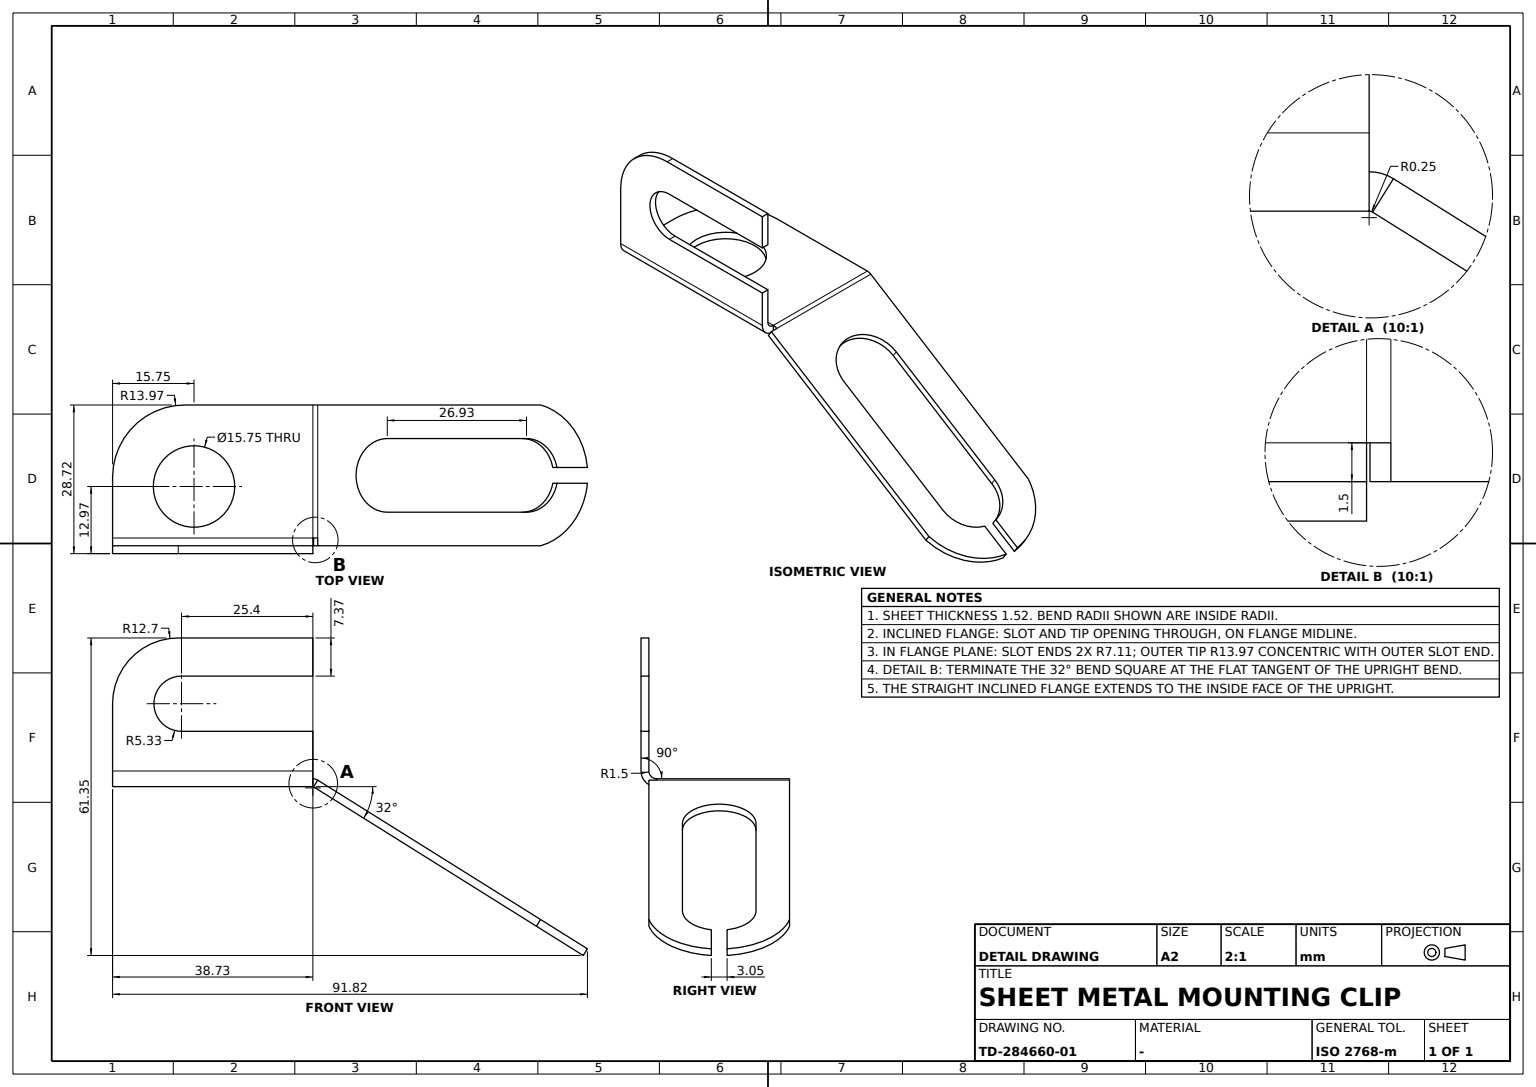
ISO-10303-21;
HEADER;
FILE_DESCRIPTION((''),'2;1');
FILE_NAME('','',(''),(''),'','','');
FILE_SCHEMA(('AUTOMOTIVE_DESIGN'));
ENDSEC;
DATA;
#1=APPLICATION_CONTEXT('');
#2=PRODUCT_CONTEXT('',#1,'mechanical');
#3=PRODUCT('','','',(#2));
#4=PRODUCT_DEFINITION_FORMATION('','',#3);
#5=PRODUCT_DEFINITION_CONTEXT('',#1,'design');
#6=PRODUCT_DEFINITION('','',#4,#5);
#7=PRODUCT_DEFINITION_SHAPE('','',#6);
#8=(LENGTH_UNIT()NAMED_UNIT(*)SI_UNIT(.MILLI.,.METRE.));
#9=(NAMED_UNIT(*)PLANE_ANGLE_UNIT()SI_UNIT($,.RADIAN.));
#10=(NAMED_UNIT(*)SI_UNIT($,.STERADIAN.)SOLID_ANGLE_UNIT());
#11=UNCERTAINTY_MEASURE_WITH_UNIT(LENGTH_MEASURE(0.005),#8,'distance_accuracy_value','');
#12=(GEOMETRIC_REPRESENTATION_CONTEXT(3)GLOBAL_UNCERTAINTY_ASSIGNED_CONTEXT((#11))GLOBAL_UNIT_ASSIGNED_CONTEXT((#8,#9,#10))REPRESENTATION_CONTEXT('',''));
#13=CARTESIAN_POINT('',(72.417726,1.524,-32.856272));
#14=VERTEX_POINT('',#13);
#15=CARTESIAN_POINT('',(63.358061,13.5977,-27.195165));
#16=VERTEX_POINT('',#15);
#17=CARTESIAN_POINT('',(60.641201,0.,-25.497482));
#18=DIRECTION('',(0.529919264,0.,0.848048096));
#19=DIRECTION('',(0.848048096,0.,-0.529919264));
#20=AXIS2_PLACEMENT_3D('',#17,#18,#19);
#21=CIRCLE('',#20,13.97);
#22=EDGE_CURVE('',#14,#16,#21,.T.);
#23=ORIENTED_EDGE('',*,*,#22,.T.);
#24=CARTESIAN_POINT('',(20.26809,13.5977,-0.269563));
#25=VERTEX_POINT('',#24);
#26=CARTESIAN_POINT('',(50.807597,13.5977,-19.352764));
#27=VECTOR('',#19,1000.);
#28=LINE('',#26,#27);
#29=EDGE_CURVE('',#25,#16,#28,.T.);
#30=ORIENTED_EDGE('',*,*,#29,.F.);
#31=CARTESIAN_POINT('',(20.26809,-12.0977,-0.269563));
#32=VERTEX_POINT('',#31);
#33=CARTESIAN_POINT('',(20.26809,0.,-0.269563));
#34=DIRECTION('',(0.,1.,0.));
#35=VECTOR('',#34,1000.);
#36=LINE('',#33,#35);
#37=EDGE_CURVE('',#32,#25,#36,.T.);
#38=ORIENTED_EDGE('',*,*,#37,.F.);
#39=CARTESIAN_POINT('',(20.26809,-13.5977,-0.269563));
#40=VERTEX_POINT('',#39);
#41=DIRECTION('',(0.,-1.,0.));
#42=VECTOR('',#41,1000.);
#43=LINE('',#33,#42);
#44=EDGE_CURVE('',#32,#40,#43,.T.);
#45=ORIENTED_EDGE('',*,*,#44,.T.);
#46=CARTESIAN_POINT('',(63.358061,-13.5977,-27.195165));
#47=VERTEX_POINT('',#46);
#48=CARTESIAN_POINT('',(50.807597,-13.5977,-19.352764));
#49=LINE('',#48,#27);
#50=EDGE_CURVE('',#40,#47,#49,.T.);
#51=ORIENTED_EDGE('',*,*,#50,.T.);
#52=CARTESIAN_POINT('',(72.417726,-1.524,-32.856272));
#53=VERTEX_POINT('',#52);
#54=EDGE_CURVE('',#47,#53,#21,.T.);
#55=ORIENTED_EDGE('',*,*,#54,.T.);
#56=CARTESIAN_POINT('',(66.532418,-1.524,-29.178723));
#57=VERTEX_POINT('',#56);
#58=CARTESIAN_POINT('',(20.207297,-1.524,-0.231575));
#59=DIRECTION('',(-0.848048096,0.,0.529919264));
#60=VECTOR('',#59,1000.);
#61=LINE('',#58,#60);
#62=EDGE_CURVE('',#53,#57,#61,.T.);
#63=ORIENTED_EDGE('',*,*,#62,.T.);
#64=CARTESIAN_POINT('',(60.641201,-7.112,-25.497482));
#65=VERTEX_POINT('',#64);
#66=CIRCLE('',#20,7.112);
#67=EDGE_CURVE('',#65,#57,#66,.T.);
#68=ORIENTED_EDGE('',*,*,#67,.F.);
#69=CARTESIAN_POINT('',(33.715674,-7.112,-8.672545));
#70=VERTEX_POINT('',#69);
#71=CARTESIAN_POINT('',(47.178437,-7.112,-17.085014));
#72=LINE('',#71,#60);
#73=EDGE_CURVE('',#65,#70,#72,.T.);
#74=ORIENTED_EDGE('',*,*,#73,.T.);
#75=CARTESIAN_POINT('',(33.715674,7.112,-8.672545));
#76=VERTEX_POINT('',#75);
#77=CARTESIAN_POINT('',(33.715674,0.,-8.672545));
#78=AXIS2_PLACEMENT_3D('',#77,#18,#19);
#79=CIRCLE('',#78,7.112);
#80=EDGE_CURVE('',#70,#76,#79,.F.);
#81=ORIENTED_EDGE('',*,*,#80,.T.);
#82=CARTESIAN_POINT('',(60.641201,7.112,-25.497482));
#83=VERTEX_POINT('',#82);
#84=CARTESIAN_POINT('',(20.207297,7.112,-0.231575));
#85=LINE('',#84,#60);
#86=EDGE_CURVE('',#83,#76,#85,.T.);
#87=ORIENTED_EDGE('',*,*,#86,.F.);
#88=CARTESIAN_POINT('',(66.532418,1.524,-29.178723));
#89=VERTEX_POINT('',#88);
#90=EDGE_CURVE('',#89,#83,#66,.T.);
#91=ORIENTED_EDGE('',*,*,#90,.F.);
#92=CARTESIAN_POINT('',(20.207297,1.524,-0.231575));
#93=LINE('',#92,#27);
#94=EDGE_CURVE('',#89,#14,#93,.T.);
#95=ORIENTED_EDGE('',*,*,#94,.T.);
#96=EDGE_LOOP('',(#23,#30,#38,#45,#51,#55,#63,#68,#74,#81,#87,#91,#95));
#97=FACE_BOUND('',#96,.T.);
#98=CARTESIAN_POINT('',(20.207297,0.,-0.231575));
#99=AXIS2_PLACEMENT_3D('',#98,#18,#19);
#100=PLANE('',#99);
#101=ADVANCED_FACE('',(#97),#100,.T.);
#102=CARTESIAN_POINT('',(59.833604,-7.112,-26.789907));
#103=VERTEX_POINT('',#102);
#104=VECTOR('',#18,1000.);
#105=LINE('',#64,#104);
#106=EDGE_CURVE('',#65,#103,#105,.F.);
#107=ORIENTED_EDGE('',*,*,#106,.F.);
#108=ORIENTED_EDGE('',*,*,#67,.T.);
#109=CARTESIAN_POINT('',(65.724821,-1.524,-30.471148));
#110=VERTEX_POINT('',#109);
#111=LINE('',#56,#104);
#112=EDGE_CURVE('',#57,#110,#111,.F.);
#113=ORIENTED_EDGE('',*,*,#112,.T.);
#114=CARTESIAN_POINT('',(59.833604,0.,-26.789907));
#115=AXIS2_PLACEMENT_3D('',#114,#18,#19);
#116=CIRCLE('',#115,7.112);
#117=EDGE_CURVE('',#103,#110,#116,.T.);
#118=ORIENTED_EDGE('',*,*,#117,.F.);
#119=EDGE_LOOP('',(#107,#108,#113,#118));
#120=FACE_BOUND('',#119,.T.);
#121=CYLINDRICAL_SURFACE('',#20,7.112);
#122=ADVANCED_FACE('',(#120),#121,.F.);
#123=CARTESIAN_POINT('',(62.550464,-13.5977,-28.48759));
#124=VERTEX_POINT('',#123);
#125=LINE('',#46,#104);
#126=EDGE_CURVE('',#47,#124,#125,.F.);
#127=ORIENTED_EDGE('',*,*,#126,.T.);
#128=CARTESIAN_POINT('',(71.610129,-1.524,-34.148697));
#129=VERTEX_POINT('',#128);
#130=CIRCLE('',#115,13.97);
#131=EDGE_CURVE('',#124,#129,#130,.T.);
#132=ORIENTED_EDGE('',*,*,#131,.T.);
#133=LINE('',#52,#104);
#134=EDGE_CURVE('',#53,#129,#133,.F.);
#135=ORIENTED_EDGE('',*,*,#134,.F.);
#136=ORIENTED_EDGE('',*,*,#54,.F.);
#137=EDGE_LOOP('',(#127,#132,#135,#136));
#138=FACE_BOUND('',#137,.T.);
#139=CYLINDRICAL_SURFACE('',#20,13.97);
#140=ADVANCED_FACE('',(#138),#139,.T.);
#141=CARTESIAN_POINT('',(-19.3997,-0.3723,0.));
#142=VERTEX_POINT('',#141);
#143=CARTESIAN_POINT('',(-5.4297,13.5977,0.));
#144=VERTEX_POINT('',#143);
#145=CARTESIAN_POINT('',(-5.4297,-0.3723,0.));
#146=DIRECTION('',(0.,0.,-1.));
#147=DIRECTION('',(-1.,0.,0.));
#148=AXIS2_PLACEMENT_3D('',#145,#146,#147);
#149=CIRCLE('',#148,13.97);
#150=EDGE_CURVE('',#142,#144,#149,.T.);
#151=ORIENTED_EDGE('',*,*,#150,.F.);
#152=CARTESIAN_POINT('',(-19.3997,-12.0977,0.));
#153=VERTEX_POINT('',#152);
#154=CARTESIAN_POINT('',(-19.3997,0.,0.));
#155=LINE('',#154,#35);
#156=EDGE_CURVE('',#153,#142,#155,.T.);
#157=ORIENTED_EDGE('',*,*,#156,.F.);
#158=CARTESIAN_POINT('',(19.328014,-12.0977,0.));
#159=VERTEX_POINT('',#158);
#160=CARTESIAN_POINT('',(-0.035843,-12.0977,0.));
#161=DIRECTION('',(1.,0.,0.));
#162=VECTOR('',#161,1000.);
#163=LINE('',#160,#162);
#164=EDGE_CURVE('',#153,#159,#163,.T.);
#165=ORIENTED_EDGE('',*,*,#164,.T.);
#166=CARTESIAN_POINT('',(19.328014,13.5977,0.));
#167=VERTEX_POINT('',#166);
#168=CARTESIAN_POINT('',(19.328014,0.,0.));
#169=LINE('',#168,#35);
#170=EDGE_CURVE('',#159,#167,#169,.T.);
#171=ORIENTED_EDGE('',*,*,#170,.T.);
#172=CARTESIAN_POINT('',(0.,13.5977,0.));
#173=LINE('',#172,#162);
#174=EDGE_CURVE('',#144,#167,#173,.T.);
#175=ORIENTED_EDGE('',*,*,#174,.F.);
#176=EDGE_LOOP('',(#151,#157,#165,#171,#175));
#177=FACE_BOUND('',#176,.T.);
#178=CARTESIAN_POINT('',(-11.5257,-2.1503,0.));
#179=VERTEX_POINT('',#178);
#180=CARTESIAN_POINT('',(-3.6517,-2.1503,0.));
#181=AXIS2_PLACEMENT_3D('',#180,#146,#147);
#182=CIRCLE('',#181,7.874);
#183=EDGE_CURVE('',#179,#179,#182,.T.);
#184=ORIENTED_EDGE('',*,*,#183,.T.);
#185=EDGE_LOOP('',(#184));
#186=FACE_BOUND('',#185,.T.);
#187=CARTESIAN_POINT('',(0.,0.,0.));
#188=AXIS2_PLACEMENT_3D('',#187,#146,#41);
#189=PLANE('',#188);
#190=ADVANCED_FACE('',(#177,#186),#189,.F.);
#191=CARTESIAN_POINT('',(-19.3997,-0.3723,-1.524));
#192=VERTEX_POINT('',#191);
#193=CARTESIAN_POINT('',(-5.4297,13.5977,-1.524));
#194=VERTEX_POINT('',#193);
#195=CARTESIAN_POINT('',(-5.4297,-0.3723,-1.524));
#196=AXIS2_PLACEMENT_3D('',#195,#146,#147);
#197=CIRCLE('',#196,13.97);
#198=EDGE_CURVE('',#192,#194,#197,.T.);
#199=ORIENTED_EDGE('',*,*,#198,.F.);
#200=VECTOR('',#146,1000.);
#201=LINE('',#141,#200);
#202=EDGE_CURVE('',#142,#192,#201,.T.);
#203=ORIENTED_EDGE('',*,*,#202,.F.);
#204=ORIENTED_EDGE('',*,*,#150,.T.);
#205=LINE('',#143,#200);
#206=EDGE_CURVE('',#144,#194,#205,.T.);
#207=ORIENTED_EDGE('',*,*,#206,.T.);
#208=EDGE_LOOP('',(#199,#203,#204,#207));
#209=FACE_BOUND('',#208,.T.);
#210=AXIS2_PLACEMENT_3D('',#145,#146,#41);
#211=CYLINDRICAL_SURFACE('',#210,13.97);
#212=ADVANCED_FACE('',(#209),#211,.T.);
#213=ORIENTED_EDGE('',*,*,#198,.T.);
#214=CARTESIAN_POINT('',(19.328014,13.5977,-1.524));
#215=VERTEX_POINT('',#214);
#216=CARTESIAN_POINT('',(0.,13.5977,-1.524));
#217=LINE('',#216,#162);
#218=EDGE_CURVE('',#194,#215,#217,.T.);
#219=ORIENTED_EDGE('',*,*,#218,.T.);
#220=CARTESIAN_POINT('',(19.328014,-12.0977,-1.524));
#221=VERTEX_POINT('',#220);
#222=CARTESIAN_POINT('',(19.328014,0.,-1.524));
#223=LINE('',#222,#35);
#224=EDGE_CURVE('',#221,#215,#223,.T.);
#225=ORIENTED_EDGE('',*,*,#224,.F.);
#226=CARTESIAN_POINT('',(-19.3997,-12.0977,-1.524));
#227=VERTEX_POINT('',#226);
#228=CARTESIAN_POINT('',(-0.035843,-12.0977,-1.524));
#229=LINE('',#228,#162);
#230=EDGE_CURVE('',#227,#221,#229,.T.);
#231=ORIENTED_EDGE('',*,*,#230,.F.);
#232=CARTESIAN_POINT('',(-19.3997,0.,-1.524));
#233=LINE('',#232,#35);
#234=EDGE_CURVE('',#227,#192,#233,.T.);
#235=ORIENTED_EDGE('',*,*,#234,.T.);
#236=EDGE_LOOP('',(#213,#219,#225,#231,#235));
#237=FACE_BOUND('',#236,.T.);
#238=CARTESIAN_POINT('',(-11.5257,-2.1503,-1.524));
#239=VERTEX_POINT('',#238);
#240=CARTESIAN_POINT('',(-3.6517,-2.1503,-1.524));
#241=AXIS2_PLACEMENT_3D('',#240,#146,#147);
#242=CIRCLE('',#241,7.874);
#243=EDGE_CURVE('',#239,#239,#242,.T.);
#244=ORIENTED_EDGE('',*,*,#243,.F.);
#245=EDGE_LOOP('',(#244));
#246=FACE_BOUND('',#245,.T.);
#247=CARTESIAN_POINT('',(0.,0.,-1.524));
#248=AXIS2_PLACEMENT_3D('',#247,#146,#41);
#249=PLANE('',#248);
#250=ADVANCED_FACE('',(#237,#246),#249,.T.);
#251=ORIENTED_EDGE('',*,*,#206,.F.);
#252=ORIENTED_EDGE('',*,*,#174,.T.);
#253=CARTESIAN_POINT('',(19.328014,13.5977,-1.774));
#254=DIRECTION('',(0.,0.,1.));
#255=AXIS2_PLACEMENT_3D('',#253,#34,#254);
#256=CIRCLE('',#255,1.774);
#257=EDGE_CURVE('',#25,#167,#256,.F.);
#258=ORIENTED_EDGE('',*,*,#257,.F.);
#259=ORIENTED_EDGE('',*,*,#29,.T.);
#260=CARTESIAN_POINT('',(62.550464,13.5977,-28.48759));
#261=VERTEX_POINT('',#260);
#262=LINE('',#15,#104);
#263=EDGE_CURVE('',#16,#261,#262,.F.);
#264=ORIENTED_EDGE('',*,*,#263,.T.);
#265=CARTESIAN_POINT('',(19.460493,13.5977,-1.561988));
#266=VERTEX_POINT('',#265);
#267=CARTESIAN_POINT('',(50.,13.5977,-20.64519));
#268=LINE('',#267,#27);
#269=EDGE_CURVE('',#266,#261,#268,.T.);
#270=ORIENTED_EDGE('',*,*,#269,.F.);
#271=CIRCLE('',#255,0.25);
#272=EDGE_CURVE('',#266,#215,#271,.F.);
#273=ORIENTED_EDGE('',*,*,#272,.T.);
#274=ORIENTED_EDGE('',*,*,#218,.F.);
#275=EDGE_LOOP('',(#251,#252,#258,#259,#264,#270,#273,#274));
#276=FACE_BOUND('',#275,.T.);
#277=CARTESIAN_POINT('',(50.403798,13.5977,-19.998977));
#278=AXIS2_PLACEMENT_3D('',#277,#34,#161);
#279=PLANE('',#278);
#280=ADVANCED_FACE('',(#276),#279,.T.);
#281=CARTESIAN_POINT('',(19.328014,-13.5977,27.1984));
#282=VERTEX_POINT('',#281);
#283=CARTESIAN_POINT('',(-6.6997,-13.5977,27.1984));
#284=VERTEX_POINT('',#283);
#285=CARTESIAN_POINT('',(50.403798,-13.5977,27.1984));
#286=VECTOR('',#147,1000.);
#287=LINE('',#285,#286);
#288=EDGE_CURVE('',#282,#284,#287,.T.);
#289=ORIENTED_EDGE('',*,*,#288,.F.);
#290=CARTESIAN_POINT('',(19.328014,-13.5977,19.8324));
#291=VERTEX_POINT('',#290);
#292=LINE('',#281,#200);
#293=EDGE_CURVE('',#282,#291,#292,.T.);
#294=ORIENTED_EDGE('',*,*,#293,.T.);
#295=CARTESIAN_POINT('',(-6.071986,-13.5977,19.8324));
#296=VERTEX_POINT('',#295);
#297=LINE('',#290,#286);
#298=EDGE_CURVE('',#291,#296,#297,.T.);
#299=ORIENTED_EDGE('',*,*,#298,.T.);
#300=CARTESIAN_POINT('',(-6.071986,-13.5977,9.1644));
#301=VERTEX_POINT('',#300);
#302=CARTESIAN_POINT('',(-6.071986,-13.5977,14.4984));
#303=AXIS2_PLACEMENT_3D('',#302,#34,#254);
#304=CIRCLE('',#303,5.334);
#305=EDGE_CURVE('',#301,#296,#304,.T.);
#306=ORIENTED_EDGE('',*,*,#305,.F.);
#307=CARTESIAN_POINT('',(19.328014,-13.5977,9.1644));
#308=VERTEX_POINT('',#307);
#309=CARTESIAN_POINT('',(50.403798,-13.5977,9.1644));
#310=LINE('',#309,#286);
#311=EDGE_CURVE('',#308,#301,#310,.T.);
#312=ORIENTED_EDGE('',*,*,#311,.F.);
#313=CARTESIAN_POINT('',(19.328014,-13.5977,1.5));
#314=VERTEX_POINT('',#313);
#315=CARTESIAN_POINT('',(19.328014,-13.5977,-19.998977));
#316=VECTOR('',#254,1000.);
#317=LINE('',#315,#316);
#318=EDGE_CURVE('',#314,#308,#317,.T.);
#319=ORIENTED_EDGE('',*,*,#318,.F.);
#320=CARTESIAN_POINT('',(-19.3997,-13.5977,1.5));
#321=VERTEX_POINT('',#320);
#322=CARTESIAN_POINT('',(-0.035843,-13.5977,1.5));
#323=LINE('',#322,#162);
#324=EDGE_CURVE('',#321,#314,#323,.T.);
#325=ORIENTED_EDGE('',*,*,#324,.F.);
#326=CARTESIAN_POINT('',(-19.3997,-13.5977,14.4984));
#327=VERTEX_POINT('',#326);
#328=CARTESIAN_POINT('',(-19.3997,-13.5977,-19.998977));
#329=LINE('',#328,#316);
#330=EDGE_CURVE('',#327,#321,#329,.F.);
#331=ORIENTED_EDGE('',*,*,#330,.F.);
#332=CARTESIAN_POINT('',(-6.6997,-13.5977,14.4984));
#333=AXIS2_PLACEMENT_3D('',#332,#34,#254);
#334=CIRCLE('',#333,12.7);
#335=EDGE_CURVE('',#284,#327,#334,.F.);
#336=ORIENTED_EDGE('',*,*,#335,.F.);
#337=EDGE_LOOP('',(#289,#294,#299,#306,#312,#319,#325,#331,#336));
#338=FACE_BOUND('',#337,.T.);
#339=CARTESIAN_POINT('',(50.403798,-13.5977,-19.998977));
#340=AXIS2_PLACEMENT_3D('',#339,#34,#161);
#341=PLANE('',#340);
#342=ADVANCED_FACE('',(#338),#341,.T.);
#343=CARTESIAN_POINT('',(19.460493,-12.0977,-1.561988));
#344=VERTEX_POINT('',#343);
#345=CARTESIAN_POINT('',(19.328014,-12.0977,-1.774));
#346=AXIS2_PLACEMENT_3D('',#345,#41,#146);
#347=CIRCLE('',#346,0.25);
#348=EDGE_CURVE('',#344,#221,#347,.T.);
#349=ORIENTED_EDGE('',*,*,#348,.T.);
#350=ORIENTED_EDGE('',*,*,#224,.T.);
#351=ORIENTED_EDGE('',*,*,#272,.F.);
#352=CARTESIAN_POINT('',(19.460493,0.,-1.561988));
#353=LINE('',#352,#35);
#354=EDGE_CURVE('',#344,#266,#353,.T.);
#355=ORIENTED_EDGE('',*,*,#354,.F.);
#356=EDGE_LOOP('',(#349,#350,#351,#355));
#357=FACE_BOUND('',#356,.T.);
#358=CARTESIAN_POINT('',(19.328014,0.,-1.774));
#359=AXIS2_PLACEMENT_3D('',#358,#34,#254);
#360=CYLINDRICAL_SURFACE('',#359,0.25);
#361=ADVANCED_FACE('',(#357),#360,.F.);
#362=LINE('',#158,#200);
#363=EDGE_CURVE('',#159,#221,#362,.T.);
#364=ORIENTED_EDGE('',*,*,#363,.T.);
#365=ORIENTED_EDGE('',*,*,#348,.F.);
#366=DIRECTION('',(-0.529919264,0.,-0.848048096));
#367=VECTOR('',#366,1000.);
#368=LINE('',#343,#367);
#369=EDGE_CURVE('',#32,#344,#368,.T.);
#370=ORIENTED_EDGE('',*,*,#369,.F.);
#371=CIRCLE('',#346,1.774);
#372=EDGE_CURVE('',#32,#159,#371,.T.);
#373=ORIENTED_EDGE('',*,*,#372,.T.);
#374=EDGE_LOOP('',(#364,#365,#370,#373));
#375=FACE_BOUND('',#374,.T.);
#376=DIRECTION('',(-0.913545458,0.,0.406736643));
#377=AXIS2_PLACEMENT_3D('',#343,#41,#376);
#378=PLANE('',#377);
#379=ADVANCED_FACE('',(#375),#378,.T.);
#380=CARTESIAN_POINT('',(19.460493,-13.5977,-1.561988));
#381=VERTEX_POINT('',#380);
#382=CARTESIAN_POINT('',(50.,-13.5977,-20.64519));
#383=LINE('',#382,#27);
#384=EDGE_CURVE('',#381,#124,#383,.T.);
#385=ORIENTED_EDGE('',*,*,#384,.T.);
#386=ORIENTED_EDGE('',*,*,#126,.F.);
#387=ORIENTED_EDGE('',*,*,#50,.F.);
#388=LINE('',#380,#367);
#389=EDGE_CURVE('',#40,#381,#388,.T.);
#390=ORIENTED_EDGE('',*,*,#389,.T.);
#391=EDGE_LOOP('',(#385,#386,#387,#390));
#392=FACE_BOUND('',#391,.T.);
#393=ADVANCED_FACE('',(#392),#341,.F.);
#394=CARTESIAN_POINT('',(19.328014,-15.1217,1.5));
#395=VERTEX_POINT('',#394);
#396=LINE('',#313,#42);
#397=EDGE_CURVE('',#314,#395,#396,.T.);
#398=ORIENTED_EDGE('',*,*,#397,.F.);
#399=ORIENTED_EDGE('',*,*,#318,.T.);
#400=CARTESIAN_POINT('',(19.328014,-15.1217,9.1644));
#401=VERTEX_POINT('',#400);
#402=LINE('',#307,#35);
#403=EDGE_CURVE('',#401,#308,#402,.T.);
#404=ORIENTED_EDGE('',*,*,#403,.F.);
#405=CARTESIAN_POINT('',(19.328014,-15.1217,0.));
#406=LINE('',#405,#316);
#407=EDGE_CURVE('',#395,#401,#406,.T.);
#408=ORIENTED_EDGE('',*,*,#407,.F.);
#409=EDGE_LOOP('',(#398,#399,#404,#408));
#410=FACE_BOUND('',#409,.T.);
#411=AXIS2_PLACEMENT_3D('',#281,#147,#146);
#412=PLANE('',#411);
#413=ADVANCED_FACE('',(#410),#412,.F.);
#414=ORIENTED_EDGE('',*,*,#243,.T.);
#415=EDGE_LOOP('',(#414));
#416=FACE_BOUND('',#415,.T.);
#417=ORIENTED_EDGE('',*,*,#183,.F.);
#418=EDGE_LOOP('',(#417));
#419=FACE_BOUND('',#418,.T.);
#420=CARTESIAN_POINT('',(-3.6517,-2.1503,-0.762));
#421=AXIS2_PLACEMENT_3D('',#420,#146,#161);
#422=CYLINDRICAL_SURFACE('',#421,7.874);
#423=ADVANCED_FACE('',(#416,#419),#422,.F.);
#424=CARTESIAN_POINT('',(65.724821,1.524,-30.471148));
#425=VERTEX_POINT('',#424);
#426=CARTESIAN_POINT('',(71.610129,1.524,-34.148697));
#427=VERTEX_POINT('',#426);
#428=CARTESIAN_POINT('',(19.3997,1.524,-1.524));
#429=LINE('',#428,#27);
#430=EDGE_CURVE('',#425,#427,#429,.T.);
#431=ORIENTED_EDGE('',*,*,#430,.T.);
#432=LINE('',#13,#104);
#433=EDGE_CURVE('',#14,#427,#432,.F.);
#434=ORIENTED_EDGE('',*,*,#433,.F.);
#435=ORIENTED_EDGE('',*,*,#94,.F.);
#436=LINE('',#88,#104);
#437=EDGE_CURVE('',#89,#425,#436,.F.);
#438=ORIENTED_EDGE('',*,*,#437,.T.);
#439=EDGE_LOOP('',(#431,#434,#435,#438));
#440=FACE_BOUND('',#439,.T.);
#441=CARTESIAN_POINT('',(69.475072,1.524,-31.017497));
#442=AXIS2_PLACEMENT_3D('',#441,#41,#161);
#443=PLANE('',#442);
#444=ADVANCED_FACE('',(#440),#443,.T.);
#445=CARTESIAN_POINT('',(-19.3997,-15.1217,1.5));
#446=VERTEX_POINT('',#445);
#447=LINE('',#320,#35);
#448=EDGE_CURVE('',#321,#446,#447,.F.);
#449=ORIENTED_EDGE('',*,*,#448,.T.);
#450=CARTESIAN_POINT('',(-19.3997,-15.1217,14.4984));
#451=VERTEX_POINT('',#450);
#452=CARTESIAN_POINT('',(-19.3997,-15.1217,0.));
#453=LINE('',#452,#316);
#454=EDGE_CURVE('',#451,#446,#453,.F.);
#455=ORIENTED_EDGE('',*,*,#454,.F.);
#456=LINE('',#326,#35);
#457=EDGE_CURVE('',#327,#451,#456,.F.);
#458=ORIENTED_EDGE('',*,*,#457,.F.);
#459=ORIENTED_EDGE('',*,*,#330,.T.);
#460=EDGE_LOOP('',(#449,#455,#458,#459));
#461=FACE_BOUND('',#460,.T.);
#462=CARTESIAN_POINT('',(-19.3997,-13.5977,0.));
#463=AXIS2_PLACEMENT_3D('',#462,#147,#34);
#464=PLANE('',#463);
#465=ADVANCED_FACE('',(#461),#464,.T.);
#466=CARTESIAN_POINT('',(-0.035843,-15.1217,1.5));
#467=LINE('',#466,#162);
#468=EDGE_CURVE('',#446,#395,#467,.T.);
#469=ORIENTED_EDGE('',*,*,#468,.T.);
#470=ORIENTED_EDGE('',*,*,#407,.T.);
#471=CARTESIAN_POINT('',(-6.071986,-15.1217,9.1644));
#472=VERTEX_POINT('',#471);
#473=CARTESIAN_POINT('',(0.,-15.1217,9.1644));
#474=LINE('',#473,#286);
#475=EDGE_CURVE('',#401,#472,#474,.T.);
#476=ORIENTED_EDGE('',*,*,#475,.T.);
#477=CARTESIAN_POINT('',(-6.071986,-15.1217,19.8324));
#478=VERTEX_POINT('',#477);
#479=CARTESIAN_POINT('',(-6.071986,-15.1217,14.4984));
#480=AXIS2_PLACEMENT_3D('',#479,#34,#254);
#481=CIRCLE('',#480,5.334);
#482=EDGE_CURVE('',#472,#478,#481,.T.);
#483=ORIENTED_EDGE('',*,*,#482,.T.);
#484=CARTESIAN_POINT('',(19.328014,-15.1217,19.8324));
#485=VERTEX_POINT('',#484);
#486=LINE('',#484,#286);
#487=EDGE_CURVE('',#485,#478,#486,.T.);
#488=ORIENTED_EDGE('',*,*,#487,.F.);
#489=CARTESIAN_POINT('',(19.328014,-15.1217,27.1984));
#490=VERTEX_POINT('',#489);
#491=LINE('',#489,#200);
#492=EDGE_CURVE('',#490,#485,#491,.T.);
#493=ORIENTED_EDGE('',*,*,#492,.F.);
#494=CARTESIAN_POINT('',(-6.6997,-15.1217,27.1984));
#495=VERTEX_POINT('',#494);
#496=CARTESIAN_POINT('',(0.,-15.1217,27.1984));
#497=LINE('',#496,#286);
#498=EDGE_CURVE('',#490,#495,#497,.T.);
#499=ORIENTED_EDGE('',*,*,#498,.T.);
#500=CARTESIAN_POINT('',(-6.6997,-15.1217,14.4984));
#501=AXIS2_PLACEMENT_3D('',#500,#34,#254);
#502=CIRCLE('',#501,12.7);
#503=EDGE_CURVE('',#495,#451,#502,.F.);
#504=ORIENTED_EDGE('',*,*,#503,.T.);
#505=ORIENTED_EDGE('',*,*,#454,.T.);
#506=EDGE_LOOP('',(#469,#470,#476,#483,#488,#493,#499,#504,#505));
#507=FACE_BOUND('',#506,.T.);
#508=CARTESIAN_POINT('',(0.,-15.1217,0.));
#509=AXIS2_PLACEMENT_3D('',#508,#34,#147);
#510=PLANE('',#509);
#511=ADVANCED_FACE('',(#507),#510,.F.);
#512=LINE('',#152,#200);
#513=EDGE_CURVE('',#153,#227,#512,.T.);
#514=ORIENTED_EDGE('',*,*,#513,.T.);
#515=CARTESIAN_POINT('',(-19.3997,-12.0977,1.5));
#516=AXIS2_PLACEMENT_3D('',#515,#161,#146);
#517=CIRCLE('',#516,3.024);
#518=EDGE_CURVE('',#446,#227,#517,.T.);
#519=ORIENTED_EDGE('',*,*,#518,.F.);
#520=ORIENTED_EDGE('',*,*,#448,.F.);
#521=CIRCLE('',#516,1.5);
#522=EDGE_CURVE('',#321,#153,#521,.T.);
#523=ORIENTED_EDGE('',*,*,#522,.T.);
#524=EDGE_LOOP('',(#514,#519,#520,#523));
#525=FACE_BOUND('',#524,.T.);
#526=CARTESIAN_POINT('',(-19.3997,-12.239072,0.));
#527=CARTESIAN_POINT('',(-19.3997,-12.382705,-1.524));
#528=CARTESIAN_POINT('',(-19.3997,-12.380443,0.016655));
#529=CARTESIAN_POINT('',(-19.3997,-12.667711,-1.490424));
#530=CARTESIAN_POINT('',(-19.3997,-12.519198,0.049967));
#531=CARTESIAN_POINT('',(-19.3997,-12.947441,-1.423266));
#532=CARTESIAN_POINT('',(-19.3997,-12.786247,0.148651));
#533=CARTESIAN_POINT('',(-19.3997,-13.485811,-1.224321));
#534=CARTESIAN_POINT('',(-19.3997,-13.023051,0.306693));
#535=CARTESIAN_POINT('',(-19.3997,-13.963207,-0.905708));
#536=CARTESIAN_POINT('',(-19.3997,-13.131559,0.399367));
#537=CARTESIAN_POINT('',(-19.3997,-14.18196,-0.718875));
#538=CARTESIAN_POINT('',(-19.3997,-13.3247,0.608533));
#539=CARTESIAN_POINT('',(-19.3997,-14.571331,-0.297198));
#540=CARTESIAN_POINT('',(-19.3997,-13.463944,0.856856));
#541=CARTESIAN_POINT('',(-19.3997,-14.852047,0.203421));
#542=CARTESIAN_POINT('',(-19.3997,-13.518552,0.988691));
#543=CARTESIAN_POINT('',(-19.3997,-14.962137,0.469202));
#544=CARTESIAN_POINT('',(-19.3997,-13.569972,1.171392));
#545=CARTESIAN_POINT('',(-19.3997,-15.065801,0.837527));
#546=CARTESIAN_POINT('',(-19.3997,-13.592148,1.358725));
#547=CARTESIAN_POINT('',(-19.3997,-15.110508,1.21519));
#548=CARTESIAN_POINT('',(-19.3997,-13.595849,1.405752));
#549=CARTESIAN_POINT('',(-19.3997,-15.117969,1.309996));
#550=CARTESIAN_POINT('',(-19.3997,-13.5977,1.452876));
#551=CARTESIAN_POINT('',(-19.3997,-15.1217,1.404998));
#552=B_SPLINE_SURFACE_WITH_KNOTS('',5,1,((#152,#226),(#526,#527),(#528,#529),(#530,#531),(#532,#533),(#534,#535),(#536,#537),(#538,#539),(#540,#541),(#542,#543),(#544,#545),(#546,#547),(#548,#549),(#550,#551),(#320,#445)),.RULED_SURF.,.F.,.F.,.F.,(6,3,3,3,6),(2,2),(0.,0.0045,0.009,0.0135,0.015),(0.,0.0015),.UNSPECIFIED.);
#553=ADVANCED_FACE('',(#525),#552,.F.);
#554=ORIENTED_EDGE('',*,*,#44,.F.);
#555=ORIENTED_EDGE('',*,*,#369,.T.);
#556=LINE('',#352,#42);
#557=EDGE_CURVE('',#344,#381,#556,.T.);
#558=ORIENTED_EDGE('',*,*,#557,.T.);
#559=ORIENTED_EDGE('',*,*,#389,.F.);
#560=EDGE_LOOP('',(#554,#555,#558,#559));
#561=FACE_BOUND('',#560,.T.);
#562=CARTESIAN_POINT('',(19.460493,-12.8477,-1.561988));
#563=AXIS2_PLACEMENT_3D('',#562,#59,#18);
#564=PLANE('',#563);
#565=ADVANCED_FACE('',(#561),#564,.T.);
#566=ORIENTED_EDGE('',*,*,#503,.F.);
#567=LINE('',#283,#35);
#568=EDGE_CURVE('',#284,#495,#567,.F.);
#569=ORIENTED_EDGE('',*,*,#568,.F.);
#570=ORIENTED_EDGE('',*,*,#335,.T.);
#571=ORIENTED_EDGE('',*,*,#457,.T.);
#572=EDGE_LOOP('',(#566,#569,#570,#571));
#573=FACE_BOUND('',#572,.T.);
#574=AXIS2_PLACEMENT_3D('',#332,#34,#147);
#575=CYLINDRICAL_SURFACE('',#574,12.7);
#576=ADVANCED_FACE('',(#573),#575,.T.);
#577=LINE('',#281,#35);
#578=EDGE_CURVE('',#490,#282,#577,.T.);
#579=ORIENTED_EDGE('',*,*,#578,.T.);
#580=ORIENTED_EDGE('',*,*,#288,.T.);
#581=ORIENTED_EDGE('',*,*,#568,.T.);
#582=ORIENTED_EDGE('',*,*,#498,.F.);
#583=EDGE_LOOP('',(#579,#580,#581,#582));
#584=FACE_BOUND('',#583,.T.);
#585=CARTESIAN_POINT('',(-19.3997,-13.5977,27.1984));
#586=AXIS2_PLACEMENT_3D('',#585,#146,#161);
#587=PLANE('',#586);
#588=ADVANCED_FACE('',(#584),#587,.F.);
#589=ORIENTED_EDGE('',*,*,#90,.T.);
#590=CARTESIAN_POINT('',(59.833604,7.112,-26.789907));
#591=VERTEX_POINT('',#590);
#592=LINE('',#82,#104);
#593=EDGE_CURVE('',#83,#591,#592,.F.);
#594=ORIENTED_EDGE('',*,*,#593,.T.);
#595=EDGE_CURVE('',#425,#591,#116,.T.);
#596=ORIENTED_EDGE('',*,*,#595,.F.);
#597=ORIENTED_EDGE('',*,*,#437,.F.);
#598=EDGE_LOOP('',(#589,#594,#596,#597));
#599=FACE_BOUND('',#598,.T.);
#600=ADVANCED_FACE('',(#599),#121,.F.);
#601=ORIENTED_EDGE('',*,*,#384,.F.);
#602=ORIENTED_EDGE('',*,*,#557,.F.);
#603=ORIENTED_EDGE('',*,*,#354,.T.);
#604=ORIENTED_EDGE('',*,*,#269,.T.);
#605=EDGE_CURVE('',#427,#261,#130,.T.);
#606=ORIENTED_EDGE('',*,*,#605,.F.);
#607=ORIENTED_EDGE('',*,*,#430,.F.);
#608=ORIENTED_EDGE('',*,*,#595,.T.);
#609=CARTESIAN_POINT('',(32.908077,7.112,-9.964971));
#610=VERTEX_POINT('',#609);
#611=CARTESIAN_POINT('',(19.3997,7.112,-1.524));
#612=LINE('',#611,#60);
#613=EDGE_CURVE('',#591,#610,#612,.T.);
#614=ORIENTED_EDGE('',*,*,#613,.T.);
#615=CARTESIAN_POINT('',(32.908077,-7.112,-9.964971));
#616=VERTEX_POINT('',#615);
#617=CARTESIAN_POINT('',(32.908077,0.,-9.964971));
#618=AXIS2_PLACEMENT_3D('',#617,#18,#19);
#619=CIRCLE('',#618,7.112);
#620=EDGE_CURVE('',#616,#610,#619,.F.);
#621=ORIENTED_EDGE('',*,*,#620,.F.);
#622=CARTESIAN_POINT('',(46.37084,-7.112,-18.377439));
#623=LINE('',#622,#60);
#624=EDGE_CURVE('',#103,#616,#623,.T.);
#625=ORIENTED_EDGE('',*,*,#624,.F.);
#626=ORIENTED_EDGE('',*,*,#117,.T.);
#627=CARTESIAN_POINT('',(19.3997,-1.524,-1.524));
#628=LINE('',#627,#60);
#629=EDGE_CURVE('',#129,#110,#628,.T.);
#630=ORIENTED_EDGE('',*,*,#629,.F.);
#631=ORIENTED_EDGE('',*,*,#131,.F.);
#632=EDGE_LOOP('',(#601,#602,#603,#604,#606,#607,#608,#614,#621,#625,#626,#630,#631));
#633=FACE_BOUND('',#632,.T.);
#634=CARTESIAN_POINT('',(19.3997,0.,-1.524));
#635=AXIS2_PLACEMENT_3D('',#634,#18,#19);
#636=PLANE('',#635);
#637=ADVANCED_FACE('',(#633),#636,.F.);
#638=ORIENTED_EDGE('',*,*,#22,.F.);
#639=ORIENTED_EDGE('',*,*,#433,.T.);
#640=ORIENTED_EDGE('',*,*,#605,.T.);
#641=ORIENTED_EDGE('',*,*,#263,.F.);
#642=EDGE_LOOP('',(#638,#639,#640,#641));
#643=FACE_BOUND('',#642,.T.);
#644=ADVANCED_FACE('',(#643),#139,.T.);
#645=LINE('',#69,#104);
#646=EDGE_CURVE('',#70,#616,#645,.F.);
#647=ORIENTED_EDGE('',*,*,#646,.F.);
#648=ORIENTED_EDGE('',*,*,#73,.F.);
#649=ORIENTED_EDGE('',*,*,#106,.T.);
#650=ORIENTED_EDGE('',*,*,#624,.T.);
#651=EDGE_LOOP('',(#647,#648,#649,#650));
#652=FACE_BOUND('',#651,.T.);
#653=AXIS2_PLACEMENT_3D('',#71,#41,#161);
#654=PLANE('',#653);
#655=ADVANCED_FACE('',(#652),#654,.F.);
#656=ORIENTED_EDGE('',*,*,#578,.F.);
#657=ORIENTED_EDGE('',*,*,#492,.T.);
#658=LINE('',#290,#35);
#659=EDGE_CURVE('',#485,#291,#658,.T.);
#660=ORIENTED_EDGE('',*,*,#659,.T.);
#661=ORIENTED_EDGE('',*,*,#293,.F.);
#662=EDGE_LOOP('',(#656,#657,#660,#661));
#663=FACE_BOUND('',#662,.T.);
#664=ADVANCED_FACE('',(#663),#412,.F.);
#665=ORIENTED_EDGE('',*,*,#659,.F.);
#666=ORIENTED_EDGE('',*,*,#487,.T.);
#667=LINE('',#295,#35);
#668=EDGE_CURVE('',#296,#478,#667,.F.);
#669=ORIENTED_EDGE('',*,*,#668,.F.);
#670=ORIENTED_EDGE('',*,*,#298,.F.);
#671=EDGE_LOOP('',(#665,#666,#669,#670));
#672=FACE_BOUND('',#671,.T.);
#673=AXIS2_PLACEMENT_3D('',#290,#254,#147);
#674=PLANE('',#673);
#675=ADVANCED_FACE('',(#672),#674,.F.);
#676=ORIENTED_EDGE('',*,*,#164,.F.);
#677=ORIENTED_EDGE('',*,*,#522,.F.);
#678=ORIENTED_EDGE('',*,*,#324,.T.);
#679=CARTESIAN_POINT('',(19.328014,-12.0977,1.5));
#680=AXIS2_PLACEMENT_3D('',#679,#161,#146);
#681=CIRCLE('',#680,1.5);
#682=EDGE_CURVE('',#159,#314,#681,.F.);
#683=ORIENTED_EDGE('',*,*,#682,.F.);
#684=EDGE_LOOP('',(#676,#677,#678,#683));
#685=FACE_BOUND('',#684,.T.);
#686=CARTESIAN_POINT('',(-0.035843,-12.0977,1.5));
#687=AXIS2_PLACEMENT_3D('',#686,#161,#146);
#688=CYLINDRICAL_SURFACE('',#687,1.5);
#689=ADVANCED_FACE('',(#685),#688,.F.);
#690=LINE('',#75,#104);
#691=EDGE_CURVE('',#76,#610,#690,.F.);
#692=ORIENTED_EDGE('',*,*,#691,.T.);
#693=ORIENTED_EDGE('',*,*,#613,.F.);
#694=ORIENTED_EDGE('',*,*,#593,.F.);
#695=ORIENTED_EDGE('',*,*,#86,.T.);
#696=EDGE_LOOP('',(#692,#693,#694,#695));
#697=FACE_BOUND('',#696,.T.);
#698=CARTESIAN_POINT('',(47.178437,7.112,-17.085014));
#699=AXIS2_PLACEMENT_3D('',#698,#34,#161);
#700=PLANE('',#699);
#701=ADVANCED_FACE('',(#697),#700,.F.);
#702=ORIENTED_EDGE('',*,*,#513,.F.);
#703=ORIENTED_EDGE('',*,*,#156,.T.);
#704=ORIENTED_EDGE('',*,*,#202,.T.);
#705=ORIENTED_EDGE('',*,*,#234,.F.);
#706=EDGE_LOOP('',(#702,#703,#704,#705));
#707=FACE_BOUND('',#706,.T.);
#708=ADVANCED_FACE('',(#707),#464,.T.);
#709=ORIENTED_EDGE('',*,*,#372,.F.);
#710=ORIENTED_EDGE('',*,*,#37,.T.);
#711=ORIENTED_EDGE('',*,*,#257,.T.);
#712=ORIENTED_EDGE('',*,*,#170,.F.);
#713=EDGE_LOOP('',(#709,#710,#711,#712));
#714=FACE_BOUND('',#713,.T.);
#715=CYLINDRICAL_SURFACE('',#359,1.774);
#716=ADVANCED_FACE('',(#714),#715,.T.);
#717=LINE('',#300,#35);
#718=EDGE_CURVE('',#301,#472,#717,.F.);
#719=ORIENTED_EDGE('',*,*,#718,.T.);
#720=ORIENTED_EDGE('',*,*,#475,.F.);
#721=ORIENTED_EDGE('',*,*,#403,.T.);
#722=ORIENTED_EDGE('',*,*,#311,.T.);
#723=EDGE_LOOP('',(#719,#720,#721,#722));
#724=FACE_BOUND('',#723,.T.);
#725=AXIS2_PLACEMENT_3D('',#300,#146,#161);
#726=PLANE('',#725);
#727=ADVANCED_FACE('',(#724),#726,.F.);
#728=ORIENTED_EDGE('',*,*,#518,.T.);
#729=ORIENTED_EDGE('',*,*,#230,.T.);
#730=CIRCLE('',#680,3.024);
#731=EDGE_CURVE('',#221,#395,#730,.F.);
#732=ORIENTED_EDGE('',*,*,#731,.T.);
#733=ORIENTED_EDGE('',*,*,#468,.F.);
#734=EDGE_LOOP('',(#728,#729,#732,#733));
#735=FACE_BOUND('',#734,.T.);
#736=CYLINDRICAL_SURFACE('',#687,3.024);
#737=ADVANCED_FACE('',(#735),#736,.T.);
#738=ORIENTED_EDGE('',*,*,#620,.T.);
#739=ORIENTED_EDGE('',*,*,#691,.F.);
#740=ORIENTED_EDGE('',*,*,#80,.F.);
#741=ORIENTED_EDGE('',*,*,#646,.T.);
#742=EDGE_LOOP('',(#738,#739,#740,#741));
#743=FACE_BOUND('',#742,.T.);
#744=CYLINDRICAL_SURFACE('',#78,7.112);
#745=ADVANCED_FACE('',(#743),#744,.F.);
#746=ORIENTED_EDGE('',*,*,#305,.T.);
#747=ORIENTED_EDGE('',*,*,#668,.T.);
#748=ORIENTED_EDGE('',*,*,#482,.F.);
#749=ORIENTED_EDGE('',*,*,#718,.F.);
#750=EDGE_LOOP('',(#746,#747,#748,#749));
#751=FACE_BOUND('',#750,.T.);
#752=AXIS2_PLACEMENT_3D('',#302,#34,#147);
#753=CYLINDRICAL_SURFACE('',#752,5.334);
#754=ADVANCED_FACE('',(#751),#753,.F.);
#755=ORIENTED_EDGE('',*,*,#363,.F.);
#756=ORIENTED_EDGE('',*,*,#682,.T.);
#757=ORIENTED_EDGE('',*,*,#397,.T.);
#758=ORIENTED_EDGE('',*,*,#731,.F.);
#759=EDGE_LOOP('',(#755,#756,#757,#758));
#760=FACE_BOUND('',#759,.T.);
#761=CARTESIAN_POINT('',(19.328014,-12.239072,0.));
#762=CARTESIAN_POINT('',(19.328014,-12.382705,-1.524));
#763=CARTESIAN_POINT('',(19.328014,-12.380443,0.016655));
#764=CARTESIAN_POINT('',(19.328014,-12.667711,-1.490424));
#765=CARTESIAN_POINT('',(19.328014,-12.519198,0.049967));
#766=CARTESIAN_POINT('',(19.328014,-12.947441,-1.423266));
#767=CARTESIAN_POINT('',(19.328014,-12.786247,0.148651));
#768=CARTESIAN_POINT('',(19.328014,-13.485811,-1.224321));
#769=CARTESIAN_POINT('',(19.328014,-13.023051,0.306693));
#770=CARTESIAN_POINT('',(19.328014,-13.963207,-0.905708));
#771=CARTESIAN_POINT('',(19.328014,-13.131559,0.399367));
#772=CARTESIAN_POINT('',(19.328014,-14.18196,-0.718875));
#773=CARTESIAN_POINT('',(19.328014,-13.3247,0.608533));
#774=CARTESIAN_POINT('',(19.328014,-14.571331,-0.297198));
#775=CARTESIAN_POINT('',(19.328014,-13.463944,0.856856));
#776=CARTESIAN_POINT('',(19.328014,-14.852047,0.203421));
#777=CARTESIAN_POINT('',(19.328014,-13.518552,0.988691));
#778=CARTESIAN_POINT('',(19.328014,-14.962137,0.469202));
#779=CARTESIAN_POINT('',(19.328014,-13.569972,1.171392));
#780=CARTESIAN_POINT('',(19.328014,-15.065801,0.837527));
#781=CARTESIAN_POINT('',(19.328014,-13.592148,1.358725));
#782=CARTESIAN_POINT('',(19.328014,-15.110508,1.21519));
#783=CARTESIAN_POINT('',(19.328014,-13.595849,1.405752));
#784=CARTESIAN_POINT('',(19.328014,-15.117969,1.309996));
#785=CARTESIAN_POINT('',(19.328014,-13.5977,1.452876));
#786=CARTESIAN_POINT('',(19.328014,-15.1217,1.404998));
#787=B_SPLINE_SURFACE_WITH_KNOTS('',5,1,((#158,#220),(#761,#762),(#763,#764),(#765,#766),(#767,#768),(#769,#770),(#771,#772),(#773,#774),(#775,#776),(#777,#778),(#779,#780),(#781,#782),(#783,#784),(#785,#786),(#313,#394)),.RULED_SURF.,.F.,.F.,.F.,(6,3,3,3,6),(2,2),(0.,0.0045,0.009,0.0135,0.015),(0.,0.0015),.UNSPECIFIED.);
#788=ADVANCED_FACE('',(#760),#787,.T.);
#789=ORIENTED_EDGE('',*,*,#62,.F.);
#790=ORIENTED_EDGE('',*,*,#134,.T.);
#791=ORIENTED_EDGE('',*,*,#629,.T.);
#792=ORIENTED_EDGE('',*,*,#112,.F.);
#793=EDGE_LOOP('',(#789,#790,#791,#792));
#794=FACE_BOUND('',#793,.T.);
#795=CARTESIAN_POINT('',(69.475072,-1.524,-31.017497));
#796=AXIS2_PLACEMENT_3D('',#795,#34,#161);
#797=PLANE('',#796);
#798=ADVANCED_FACE('',(#794),#797,.T.);
#799=CLOSED_SHELL('',(#101,#122,#140,#190,#212,#250,#280,#342,#361,#379,#393,#413,#423,#444,#465,#511,#553,#565,#576,#588,#600,#637,#644,#655,#664,#675,#689,#701,#708,#716,#727,#737,#745,#754,#788,#798));
#800=MANIFOLD_SOLID_BREP('',#799);
#801=ADVANCED_BREP_SHAPE_REPRESENTATION('',(#800),#12);
#802=SHAPE_DEFINITION_REPRESENTATION(#7,#801);
ENDSEC;
END-ISO-10303-21;
